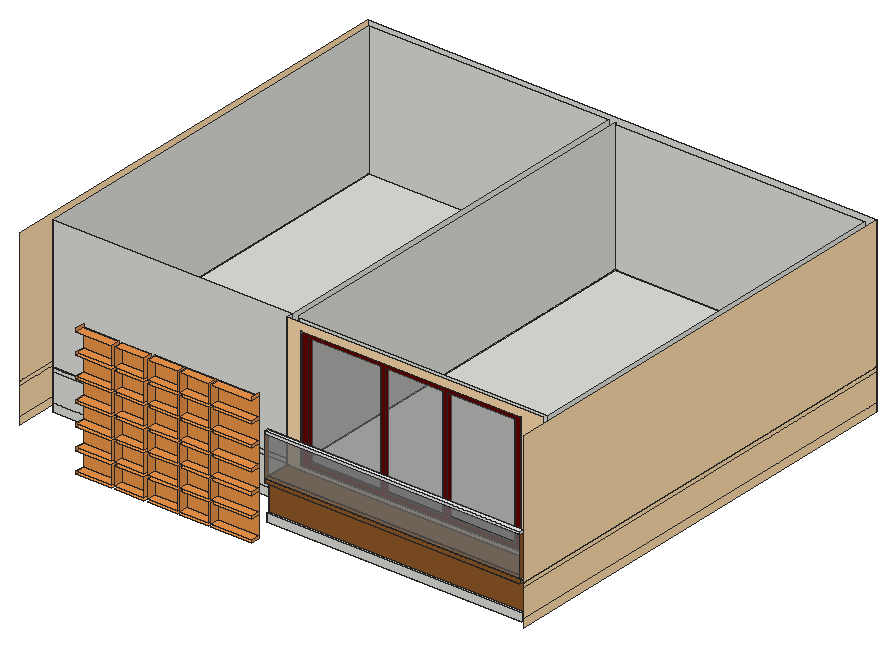
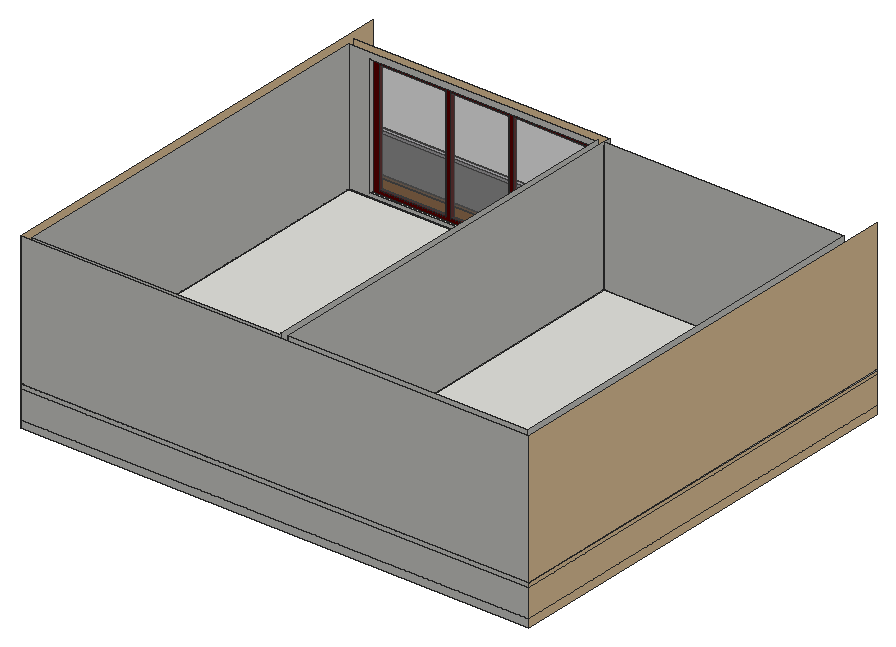
# SketchUp Ruby script. Lengths in inches.
U = 1.inch
M = Sketchup.active_model
def pt(a) = Geom::Point3d.new(a.map { |v| v * U })
def face(e, loops, mat)
  f = e.add_face(loops[0].map { |a| pt(a) })
  loops[1..].each { |l| e.add_face(l.map { |a| pt(a) }).erase! }
  f.material = f.back_material = mat if mat
  f
end
# faces: each face lists its corners as indices into pts; further lists are holes
def faces(e, pts, list, mat = nil) = list.each { |f| face(e, (f[0].is_a?(Array) ? f : [f]).map { |l| l.map { |i| pts[i] } }, mat) }
# xy, xz, yz: faces in a plane at the given z, y or x. An outline is a flat list of corners, or four numbers for a rectangle; further outlines are holes
def ring(l) = l.size == 4 ? [[l[0], l[1]], [l[2], l[1]], [l[2], l[3]], [l[0], l[3]]] : l.each_slice(2).to_a
def flat(e, list, mat, &to3) = list.each { |f| face(e, (f[0].is_a?(Array) ? f : [f]).map { |l| ring(l).map { |u, v| to3.(u, v) } }, mat) }
def xy(e, z, list, mat = nil) = flat(e, list, mat) { |x, y| [x, y, z] }
def xz(e, y, list, mat = nil) = flat(e, list, mat) { |x, z| [x, y, z] }
def yz(e, x, list, mat = nil) = flat(e, list, mat) { |y, z| [x, y, z] }
def lines(e, pts, list) = list.each { |a, b| e.add_line(pt(pts[a]), pt(pts[b])) }
# prism: a flat outline (further loops are holes) pulled along v
def prism(e, loops, v, mat = nil)
  f = face(e, loops, mat); d = Geom::Vector3d.new(v.map { |x| x * U })
  f.pushpull(f.normal.samedirection?(d) ? d.length : -d.length)
end
def box(e, o, s, mat = nil) = prism(e, [[o, [o[0] + s[0], o[1], o[2]], [o[0] + s[0], o[1] + s[1], o[2]], [o[0], o[1] + s[1], o[2]]]], [0, 0, s[2]], mat)
def at(x, y, z, deg = 0) = Geom::Transformation.translation(pt([x, y, z])) * Geom::Transformation.rotation(ORIGIN, Z_AXIS, deg.degrees)
def axes(o, x, y, z) = Geom::Transformation.new([*x, 0, *y, 0, *z, 0, *pt(o).to_a, 1])
def part(name) = M.definitions.add(name)
# library, detail: a bought-in or finely detailed component or shape, given as its bounding box
def library(name, o, s) = part(name).tap { |d| box(d.entities, o, s) }
def detail(e, o, s) = box(e.add_group.entities, o, s)
def put(e, d, t, mat = nil) = e.add_instance(d, t).tap { |i| i.material = mat if mat }
def group(e, t, mat = nil) = e.add_group.tap { |g| g.transformation = t; g.material = mat if mat }.entities
root = M.entities
M.materials.add("[0033_NavajoWhite]").color = [255, 222, 173]
M.materials.add("[Color A08]").color = [102, 0, 0]
M.materials.add("[Color M00]").color = [255, 255, 255]
M.materials.add("[Metal Silver]").color = [234, 233, 238]
M.materials.add("[Translucent Glass Gray]").color = [128, 128, 128]
M.materials["[Translucent Glass Gray]"].alpha = 0.5
M.materials.add("[Wood Floor Parquet]").color = [145, 89, 39]
M.materials.add("[Wood OSB]").color = [240, 151, 74]
c1 = part("Group\#1")
xy(c1.entities,0,[[0,0,47.4375,3.5]],"[Color A08]")
xy(c1.entities,1.52,[[1.52,0,17.01,3.5],[17.01,0,18.02,3.5],[18.02,0,30.51,3.5],[30.51,0,31.52,3.5],[31.52,0,45.92,3.5]],"[Color A08]")
xy(c1.entities,45.92,[[1.52,0,17.01,3.5],[18.02,0,30.51,3.5],[31.52,0,45.92,3.5]],"[Color A08]")
xy(c1.entities,47.4375,[[0,0,47.4375,3.5]],"[Color A08]")
xz(c1.entities,0,[[[0,0,47.4375,47.4375],[1.52,1.52,1.52,45.92,17.01,45.92,17.01,1.52,18.02,1.52,18.02,45.92,30.51,45.92,30.51,1.52,31.52,1.52,31.52,45.92,45.92,45.92,45.92,1.52]]],"[Color A08]")
xz(c1.entities,3.5,[[[0,0,47.4375,47.4375],[1.52,1.52,45.92,1.52,45.92,45.92,31.52,45.92,31.52,1.52,30.51,1.52,30.51,45.92,18.02,45.92,18.02,1.52,17.01,1.52,17.01,45.92,1.52,45.92]]],"[Color A08]")
xz(c1.entities,3.5,[[1.52,1.52,17.01,45.92],[18.02,1.52,30.51,45.92],[31.52,1.52,45.92,45.92]],"[Translucent Glass Gray]")
yz(c1.entities,0,[[0,0,3.5,47.4375]],"[Color A08]")
yz(c1.entities,1.52,[[0,1.52,3.5,45.92]],"[Color A08]")
yz(c1.entities,17.01,[[0,1.52,3.5,45.92]],"[Color A08]")
yz(c1.entities,18.02,[[0,1.52,3.5,45.92]],"[Color A08]")
yz(c1.entities,30.51,[[0,1.52,3.5,45.92]],"[Color A08]")
yz(c1.entities,31.52,[[0,1.52,3.5,45.92]],"[Color A08]")
yz(c1.entities,45.92,[[0,1.52,3.5,45.92]],"[Color A08]")
yz(c1.entities,47.4375,[[0,0,3.5,47.4375]],"[Color A08]")
xy(root,236.84,[[104.2,92.4375,136.74,100.4375],[139.19,92.4375,165.875,100.4375],[169.17,92.4375,195.99,100.4375],[198.13,92.4375,224.24,100.4375],[226.62,92.4375,263.87,100.4375]],"[Wood OSB]")
xy(root,239.48,[[104.2,92.4375,136.74,100.4375],[139.19,92.4375,165.875,100.4375],[169.17,92.4375,195.99,100.4375],[198.13,92.4375,224.24,100.4375],[226.62,92.4375,263.87,100.4375]],"[Wood OSB]")
xy(root,256.15,[[104.2,92.4375,136.74,100.4375],[139.19,92.4375,165.875,100.4375],[169.17,92.4375,195.99,100.4375],[198.13,92.4375,224.24,100.4375],[226.62,92.4375,263.87,100.4375]],"[Wood OSB]")
xy(root,258.8,[[104.2,92.4375,136.74,100.4375],[139.19,92.4375,165.875,100.4375],[169.17,92.4375,195.99,100.4375],[198.13,92.4375,224.24,100.4375],[226.62,92.4375,263.87,100.4375]],"[Wood OSB]")
xy(root,265.4375,[[304.95,100.4375,509.02,106.4375]])
xy(root,270,[[289.0625,77,521.3125,100.4375]])
xy(root,275.47,[[104.2,92.4375,136.74,100.4375],[139.19,92.4375,165.875,100.4375],[169.17,92.4375,195.99,100.4375],[198.13,92.4375,224.24,100.4375],[226.62,92.4375,263.87,100.4375]],"[Wood OSB]")
xy(root,277,[[289.0625,77,521.3125,79.6875]])
xy(root,278.11,[[104.2,92.4375,136.74,100.4375],[139.19,92.4375,165.875,100.4375],[169.17,92.4375,195.99,100.4375],[198.13,92.4375,224.24,100.4375],[226.62,92.4375,263.87,100.4375]],"[Wood OSB]")
xy(root,294.78,[[104.2,92.4375,136.74,100.4375],[139.19,92.4375,165.875,100.4375],[169.17,92.4375,195.99,100.4375],[198.13,92.4375,224.24,100.4375],[226.62,92.4375,263.87,100.4375]],"[Wood OSB]")
xy(root,297.42,[[104.2,92.4375,136.74,100.4375],[139.19,92.4375,165.875,100.4375],[169.17,92.4375,195.99,100.4375],[198.13,92.4375,224.24,100.4375],[226.62,92.4375,263.87,100.4375]],"[Wood OSB]")
xy(root,302.125,[[289.0625,74.75,521.3125,79.6875]],"[Wood Floor Parquet]")
xy(root,306,[[289.0625,74.75,521.3125,78.69],[289.0625,78.69,521.3125,100.4375]],"[Wood Floor Parquet]")
xy(root,306.125,[[71.75,106.4375,289.0625,465.125],[295.0625,106.4375,521.3125,465.125]])
xy(root,309.85,[[302.01,100.4375,501.57,106.4375]])
xy(root,314.09,[[104.2,92.4375,136.74,100.4375],[139.19,92.4375,165.875,100.4375],[169.17,92.4375,195.99,100.4375],[198.13,92.4375,224.24,100.4375],[226.62,92.4375,263.87,100.4375]],"[Wood OSB]")
xy(root,316.73,[[104.2,92.4375,136.74,100.4375],[139.19,92.4375,165.875,100.4375],[169.17,92.4375,195.99,100.4375],[198.13,92.4375,224.24,100.4375],[226.62,92.4375,263.87,100.4375]],"[Wood OSB]")
xy(root,333.4,[[104.2,92.4375,136.74,100.4375],[139.19,92.4375,165.875,100.4375],[169.17,92.4375,195.99,100.4375],[198.13,92.4375,224.24,100.4375],[226.62,92.4375,263.87,100.4375]],"[Wood OSB]")
xy(root,336.05,[[104.2,92.4375,136.74,100.4375],[139.19,92.4375,165.875,100.4375],[169.17,92.4375,195.99,100.4375],[198.13,92.4375,224.24,100.4375],[226.62,92.4375,263.87,100.4375]],"[Wood OSB]")
xy(root,342,[[289.0625,74.75,521.3125,78.69]],"[Metal Silver]")
xy(root,344.375,[[289.0625,74.75,521.3125,78.69]],"[Metal Silver]")
xy(root,352.72,[[104.2,92.4375,136.74,100.4375],[139.19,92.4375,165.875,100.4375],[169.17,92.4375,195.99,100.4375],[198.13,92.4375,224.24,100.4375],[226.62,92.4375,263.87,100.4375]],"[Wood OSB]")
xz(root,74.75,[[289.0625,342,521.3125,344.375]],"[Metal Silver]")
xz(root,74.75,[[289.0625,306,521.3125,342]],"[Translucent Glass Gray]")
xz(root,74.75,[[289.0625,302.125,521.3125,306]],"[Wood Floor Parquet]")
xz(root,77,[[289.0625,270,521.3125,277]])
xz(root,78.69,[[289.0625,342,521.3125,344.375]],"[Metal Silver]")
xz(root,78.69,[[289.0625,306,521.3125,342]],"[Translucent Glass Gray]")
xz(root,79.6875,[[289.0625,277,521.3125,302.125]],"[Wood Floor Parquet]")
xz(root,100.4375,[[289.0625,306,521.3125,306.0625],[289.0625,306.0625,521.3125,306.125]])
xz(root,100.4375,[[[289.0625,306.125,521.3125,426.125],[302.01,309.85,501.57,419.04]]],"[0033_NavajoWhite]")
xz(root,100.4375,[[104.2,239.48,136.74,256.15],[139.19,239.48,165.875,256.15],[169.17,239.48,195.99,256.15],[198.13,239.48,224.24,256.15],[226.62,239.48,263.87,256.15],
  [104.2,258.8,136.74,275.47],[139.19,258.8,165.875,275.47],[169.17,258.8,195.99,275.47],[198.13,258.8,224.24,275.47],[226.62,258.8,263.87,275.47],
  [104.2,278.11,136.74,294.78],[139.19,278.11,165.875,294.78],[169.17,278.11,195.99,294.78],[198.13,278.11,224.24,294.78],[226.62,278.11,263.87,294.78],
  [104.2,297.42,136.74,314.09],[139.19,297.42,165.875,314.09],[169.17,297.42,195.99,314.09],[198.13,297.42,224.24,314.09],[226.62,297.42,263.87,314.09],
  [104.2,316.73,136.74,333.4],[139.19,316.73,165.875,333.4],[169.17,316.73,195.99,333.4],[198.13,316.73,224.24,333.4],[226.62,316.73,263.87,333.4],
  [104.2,336.05,136.74,352.72],[139.19,336.05,165.875,352.72],[169.17,336.05,195.99,352.72],[198.13,336.05,224.24,352.72],[226.62,336.05,263.87,352.72]],"[Wood OSB]")
xz(root,106.4375,[[71.75,270,289.0625,277],[295.0625,270,521.3125,277],[71.75,277,289.0625,302.125],[295.0625,277,521.3125,302.125],[71.75,302.125,289.0625,306],
  [295.0625,302.125,521.3125,306],[71.75,306,289.0625,306.0625],[295.0625,306,521.3125,306.0625],[71.75,306.0625,289.0625,306.125],[295.0625,306.0625,521.3125,306.125],
  [71.75,306.125,289.0625,426.125],[[295.0625,306.125,295.0625,426.125,295.25,426.125,295.25,424.5,521.3125,424.5,521.3125,306.125],[302.01,309.85,501.57,419.04]]])
xz(root,465.125,[[71.75,270,289.0625,277],[295.0625,270,521.3125,277],[71.75,277,289.0625,302.125],[295.0625,277,521.3125,302.125],[71.75,302.125,289.0625,306],
  [295.0625,302.125,521.3125,306],[295.0625,306,521.3125,306.0625],[295.0625,306.0625,521.3125,306.125],[71.75,306.125,289.0625,426.125],[295.0625,306.125,521.3125,306.125,521.3125,424.5,295.25,424.5,295.25,426.125,295.0625,426.125]])
xz(root,465.125,[[71.75,306,289.0625,306.125]],"[Color M00]")
xz(root,471.125,[[65.75,270,527.3125,277],[65.75,277,527.3125,302.125],[65.75,302.125,527.3125,306],[65.75,306,527.3125,306.0625],[65.75,306.0625,527.3125,306.125],
  [65.75,306.125,527.3125,426.125]])
yz(root,65.75,[[77,306,471.125,306.0625],[77,306.0625,471.125,306.125]])
yz(root,65.75,[[77,270,471.125,277],[77,277,471.125,302.125],[77,302.125,471.125,306],[77,306.125,471.125,426.125]],"[0033_NavajoWhite]")
yz(root,71.75,[[106.4375,270,465.125,277],[106.4375,277,465.125,302.125],[106.4375,302.125,465.125,306],[106.4375,306.125,465.125,426.125]])
yz(root,71.75,[[106.4375,306,465.125,306.125]],"[Color M00]")
yz(root,104.2,[[92.4375,236.84,100.4375,239.48],[92.4375,256.15,100.4375,258.8],[92.4375,275.47,100.4375,278.11],[92.4375,294.78,100.4375,297.42],[92.4375,314.09,100.4375,316.73],
  [92.4375,333.4,100.4375,336.05],[92.4375,352.72,100.4375,355.36]],"[Wood OSB]")
yz(root,136.74,[[92.4375,239.48,100.4375,256.15],[92.4375,258.8,100.4375,275.47],[92.4375,278.11,100.4375,294.78],[92.4375,297.42,100.4375,314.09],[92.4375,316.73,100.4375,333.4],
  [92.4375,336.05,100.4375,352.72]],"[Wood OSB]")
yz(root,139.19,[[92.4375,239.48,100.4375,256.15],[92.4375,258.8,100.4375,275.47],[92.4375,278.11,100.4375,294.78],[92.4375,297.42,100.4375,314.09],[92.4375,316.73,100.4375,333.4],
  [92.4375,336.05,100.4375,352.72]],"[Wood OSB]")
yz(root,165.875,[[92.4375,239.48,100.4375,256.15],[92.4375,258.8,100.4375,275.47],[92.4375,278.11,100.4375,294.78],[92.4375,297.42,100.4375,314.09],[92.4375,316.73,100.4375,333.4],
  [92.4375,336.05,100.4375,352.72]],"[Wood OSB]")
yz(root,169.17,[[92.4375,239.48,100.4375,256.15],[92.4375,258.8,100.4375,275.47],[92.4375,278.11,100.4375,294.78],[92.4375,297.42,100.4375,314.09],[92.4375,316.73,100.4375,333.4],
  [92.4375,336.05,100.4375,352.72]],"[Wood OSB]")
yz(root,195.99,[[92.4375,239.48,100.4375,256.15],[92.4375,258.8,100.4375,275.47],[92.4375,278.11,100.4375,294.78],[92.4375,297.42,100.4375,314.09],[92.4375,316.73,100.4375,333.4],
  [92.4375,336.05,100.4375,352.72]],"[Wood OSB]")
yz(root,198.13,[[92.4375,239.48,100.4375,256.15],[92.4375,258.8,100.4375,275.47],[92.4375,278.11,100.4375,294.78],[92.4375,297.42,100.4375,314.09],[92.4375,316.73,100.4375,333.4],
  [92.4375,336.05,100.4375,352.72]],"[Wood OSB]")
yz(root,224.24,[[92.4375,239.48,100.4375,256.15],[92.4375,258.8,100.4375,275.47],[92.4375,278.11,100.4375,294.78],[92.4375,297.42,100.4375,314.09],[92.4375,316.73,100.4375,333.4],
  [92.4375,336.05,100.4375,352.72]],"[Wood OSB]")
yz(root,226.62,[[92.4375,239.48,100.4375,256.15],[92.4375,258.8,100.4375,275.47],[92.4375,278.11,100.4375,294.78],[92.4375,297.42,100.4375,314.09],[92.4375,316.73,100.4375,333.4],
  [92.4375,336.05,100.4375,352.72]],"[Wood OSB]")
yz(root,263.87,[[92.4375,236.84,100.4375,239.48],[92.4375,256.15,100.4375,258.8],[92.4375,275.47,100.4375,278.11],[92.4375,294.78,100.4375,297.42],[92.4375,314.09,100.4375,316.73],
  [92.4375,333.4,100.4375,336.05],[92.4375,352.72,100.4375,355.36]],"[Wood OSB]")
yz(root,289.0625,[[77,270,106.4375,277],[106.4375,270,465.125,277],[79.6875,277,106.4375,302.125],[106.4375,277,465.125,302.125],[74.75,302.125,106.4375,306],
  [106.4375,302.125,465.125,306],[100.4375,306,106.4375,306.0625],[106.4375,306,465.125,306.0625],[100.4375,306.0625,106.4375,306.125],[106.4375,306.0625,465.125,306.125],
  [100.4375,306.125,106.4375,426.125],[106.4375,306.125,465.125,426.125]])
yz(root,289.0625,[[74.75,342,78.69,344.375]],"[Metal Silver]")
yz(root,289.0625,[[74.75,306,78.69,342]],"[Wood Floor Parquet]")
yz(root,295.0625,[[106.4375,270,465.125,277],[106.4375,277,465.125,302.125],[106.4375,302.125,465.125,306],[106.4375,306,465.125,306.0625],[106.4375,306.0625,465.125,306.125],
  [106.4375,306.125,465.125,426.125]])
yz(root,302.01,[[100.4375,309.85,106.4375,419.04]])
yz(root,501.57,[[100.4375,309.85,106.4375,419.04]])
yz(root,521.3125,[[106.4375,270,465.125,277],[106.4375,277,465.125,302.125],[106.4375,302.125,465.125,306],[106.4375,306,465.125,306.0625],[106.4375,306.0625,465.125,306.125],
  [106.4375,306.125,465.125,424.5]])
yz(root,521.3125,[[74.75,342,78.69,344.375]],"[Metal Silver]")
yz(root,521.3125,[[74.75,306,78.69,342]],"[Wood Floor Parquet]")
yz(root,527.3125,[[71.3125,306,471.125,306.0625],[71.3125,306.0625,471.125,306.125]])
yz(root,527.3125,[[71.3125,270,471.125,277],[71.3125,277,471.125,302.125],[71.3125,302.125,471.125,306],[71.3125,306.125,471.125,426.125]],"[0033_NavajoWhite]")
put(root,c1,axes([302.01,101.02,309.85],[4.20685,0,0],[0,0.8342,0],[0,0,2.30171]))
